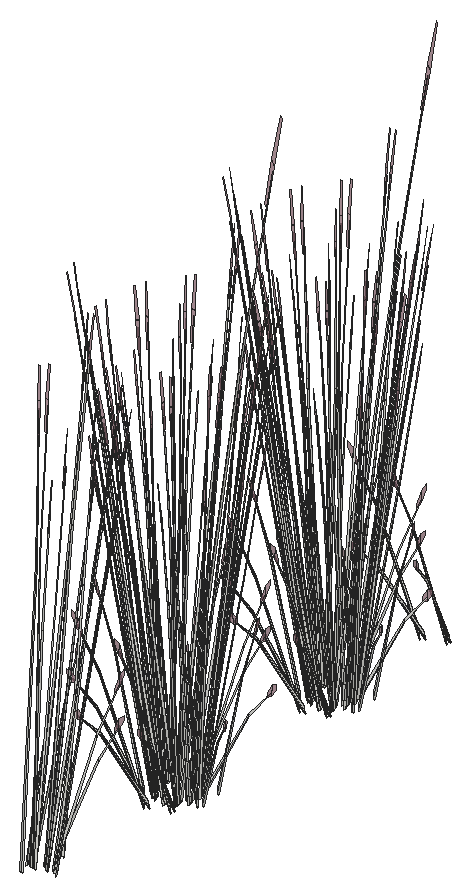
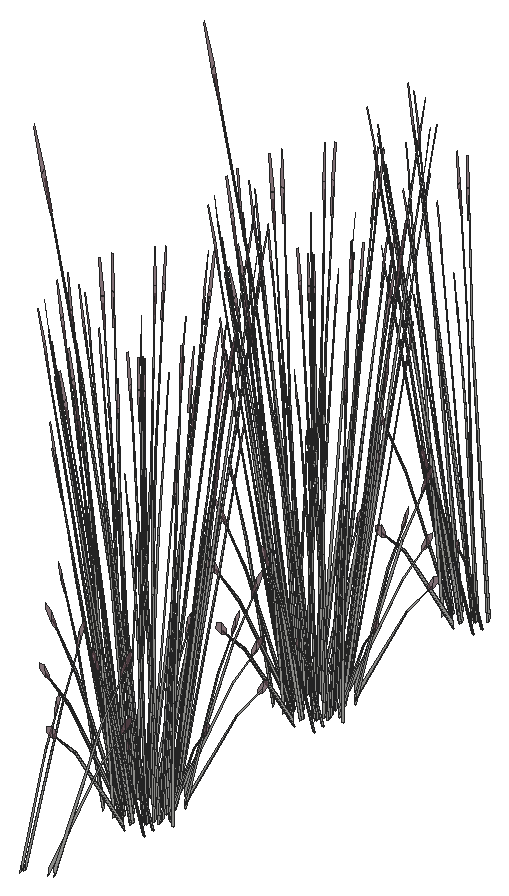
# SketchUp Ruby script. Lengths in inches.
U = 1.inch
M = Sketchup.active_model
def pt(a) = Geom::Point3d.new(a.map { |v| v * U })
def face(e, loops, mat)
  f = e.add_face(loops[0].map { |a| pt(a) })
  loops[1..].each { |l| e.add_face(l.map { |a| pt(a) }).erase! }
  f.material = f.back_material = mat if mat
  f
end
# faces: each face lists its corners as indices into pts; further lists are holes
def faces(e, pts, list, mat = nil) = list.each { |f| face(e, (f[0].is_a?(Array) ? f : [f]).map { |l| l.map { |i| pts[i] } }, mat) }
# xy, xz, yz: faces in a plane at the given z, y or x. An outline is a flat list of corners, or four numbers for a rectangle; further outlines are holes
def ring(l) = l.size == 4 ? [[l[0], l[1]], [l[2], l[1]], [l[2], l[3]], [l[0], l[3]]] : l.each_slice(2).to_a
def flat(e, list, mat, &to3) = list.each { |f| face(e, (f[0].is_a?(Array) ? f : [f]).map { |l| ring(l).map { |u, v| to3.(u, v) } }, mat) }
def xy(e, z, list, mat = nil) = flat(e, list, mat) { |x, y| [x, y, z] }
def xz(e, y, list, mat = nil) = flat(e, list, mat) { |x, z| [x, y, z] }
def yz(e, x, list, mat = nil) = flat(e, list, mat) { |y, z| [x, y, z] }
def lines(e, pts, list) = list.each { |a, b| e.add_line(pt(pts[a]), pt(pts[b])) }
# prism: a flat outline (further loops are holes) pulled along v
def prism(e, loops, v, mat = nil)
  f = face(e, loops, mat); d = Geom::Vector3d.new(v.map { |x| x * U })
  f.pushpull(f.normal.samedirection?(d) ? d.length : -d.length)
end
def box(e, o, s, mat = nil) = prism(e, [[o, [o[0] + s[0], o[1], o[2]], [o[0] + s[0], o[1] + s[1], o[2]], [o[0], o[1] + s[1], o[2]]]], [0, 0, s[2]], mat)
def at(x, y, z, deg = 0) = Geom::Transformation.translation(pt([x, y, z])) * Geom::Transformation.rotation(ORIGIN, Z_AXIS, deg.degrees)
def axes(o, x, y, z) = Geom::Transformation.new([*x, 0, *y, 0, *z, 0, *pt(o).to_a, 1])
def part(name) = M.definitions.add(name)
# library, detail: a bought-in or finely detailed component or shape, given as its bounding box
def library(name, o, s) = part(name).tap { |d| box(d.entities, o, s) }
def detail(e, o, s) = box(e.add_group.entities, o, s)
def put(e, d, t, mat = nil) = e.add_instance(d, t).tap { |i| i.material = mat if mat }
def group(e, t, mat = nil) = e.add_group.tap { |g| g.transformation = t; g.material = mat if mat }.entities
root = M.entities
M.materials.add("LightPink_Translucent").color = [144, 107, 117]
M.materials["LightPink_Translucent"].alpha = 0.75
c1 = part("blade")
p = [[2.15,0.21,22],[0,0.17,0],[0.09,0.45,0],[2.18,0.31,22],[2.29,0.31,22],[0.38,0.45,0],
  [2.48,0.24,33],[2.49,0.24,33],[2.48,0.22,33]]
faces(c1.entities,p,[[0,1,2,3],[4,5,2,3],[6,3,4,7],[8,0,3,6]])
c2 = part("seeds")
p = [[0.3,-0.1,1.38],[-0.01,-0.03,1.59],[-0.01,-0.03,0.03],[0.14,-0.07,-0.07],[0.29,-0.03,3],[0.15,0.01,3.11]]
faces(c2.entities,p,[[0,1,2,3],[1,0,4,5]],"LightPink_Translucent")
c3 = part("blade with seeds")
put(c3.entities,c1,at(0,0,0))
put(c3.entities,c2,axes([2.4,0.25,30.99],[1.5799,-0.05474,1.17369],[-0.12525,1.92788,0.29478],[-0.07173,-0.02425,1.56792]))
put(root,c3,axes([400.53,708.79,5.03],[0.32648,0.25715,-0.1216],[-0.18809,0.3724,-0.67495],[-0.09224,0.12945,1.02557]))
put(root,c3,axes([402.49,710.13,5.03],[0.21031,-0.39918,-0.1216],[0.30457,0.22997,-0.67495],[0.10587,0.11278,1.02557]))
put(root,c3,axes([401.1,709.59,5.05],[0.23881,-0.24554,0.35414],[0.22606,0.28036,-0.4572],[-0.0344,0.14245,0.87481]))
put(root,c3,axes([402.21,710.46,4.71],[0.00104,-0.05646,1.77383],[0.30246,-0.2491,-0.16761],[0.10506,0.08891,0.31391]))
put(root,c3,axes([400.88,709.8125,4.73],[-0.29004,-0.02173,0.0643],[0.00795,-0.32812,0.50621],[-0.03035,0.12569,0.77189]))
put(root,c3,axes([400.98,709.84,4.73],[-0.25132,-0.3182,0.48003],[0.2669,-0.27442,0.3958],[-0.04636,0.14929,0.9933]))
put(root,c3,axes([401.77,709.99,5.05],[0.1064,-0.35863,0.35414],[0.31043,0.1046,-0.4572],[0.02846,0.14439,0.87481]))
put(root,c3,axes([402.56,710.27,4.73],[-0.16041,0.29625,0.0643],[-0.22843,-0.17248,0.50621],[0.07385,0.09498,0.77189]))
put(root,c3,axes([402.1875,711.27,5.65],[0.2439,-0.26754,-0.06488],[0.22348,0.29302,-0.29416],[0.01573,0.08303,0.97024]))
put(root,c3,axes([402.63,710.19,4.73],[-0.35104,0.10702,0.48003],[-0.06092,-0.41983,0.3958],[0.08256,0.12373,0.9933]))
put(root,c3,axes([401.67,710.32,4.73],[-0.26007,0.1585,0.0643],[-0.12729,-0.28902,0.50621],[0.02512,0.1274,0.77189]))
put(root,c3,axes([400.15,709.86,4.72],[-0.00877,0.09229,1.74944],[0.24897,0.32105,-0.27667],[-0.06518,0.15182,0.14031]))
put(root,c3,axes([400.95,709.66,5.4],[0.3879,0.02311,-0.13498],[-0.0106,0.43749,-0.74919],[-0.02694,0.1685,1.13838]))
put(root,c3,axes([401.67,710.14,5.03],[0.34538,-0.21713,-0.1216],[0.16972,0.38536,-0.67495],[0.04557,0.16239,1.02557]))
put(root,c3,axes([401.77,710.29,5.0625],[-0.34777,-0.12192,0.53283],[0.11892,-0.40083,0.43934],[0.0209,0.15763,1.10256]))
put(root,c3,axes([400.125,710.81,4.71],[0.04004,-0.02816,1.77383],[0.33095,0.18728,-0.16761],[-0.00778,0.15594,0.31391]))
put(root,c3,axes([401.58,711.01,4.72],[0.04474,0.0751,1.74944],[0.36104,0.0295,-0.27667],[0.03631,0.16562,0.14031]))
put(root,c3,axes([401.89,721.48,4.72],[-0.05398,-0.06539,1.74944],[-0.36026,0.04145,-0.27667],[-0.0575,-0.15639,0.14031]))
put(root,c3,axes([403.51,722.29,4.72],[-0.00341,-0.09282,1.74944],[-0.28775,-0.26825,-0.27667],[0.04449,-0.16261,0.14031]))
put(root,c3,axes([403.43,721.95,4.71],[-0.03584,0.03562,1.77383],[-0.35118,-0.12018,-0.16761],[-0.01271,-0.15545,0.31391]))
put(root,c3,axes([401.52,721.27,4.71],[-0.00658,0.0559,1.77383],[-0.32474,0.20287,-0.16761],[-0.09556,-0.1037,0.31391]))
put(root,c3,axes([401.45,722.26,5.09],[0.39316,-0.11987,0.53763],[0.06823,0.47021,0.4433],[-0.09247,-0.13858,1.11249]))
put(root,c3,axes([402.34,722.35,4.73],[0.34777,0.12192,0.48003],[-0.11892,0.40083,0.3958],[-0.0209,-0.15763,0.9933]))
put(root,c3,axes([402.4375,722.49,5.03],[-0.34538,0.21713,-0.1216],[-0.16972,-0.38536,-0.67495],[-0.04557,-0.16239,1.02557]))
put(root,c3,axes([403.15,722.98,5.03],[-0.3879,-0.02311,-0.1216],[0.0106,-0.43749,-0.67495],[0.02694,-0.1685,1.02557]))
put(root,c3,axes([402.43,722.32,4.73],[0.26007,-0.1585,0.0643],[0.12729,0.28902,0.50621],[-0.02512,-0.1274,0.77189]))
put(root,c3,axes([401.54,722.36,4.73],[0.16041,-0.29625,0.0643],[0.22843,0.17248,0.50621],[-0.07385,-0.09498,0.77189]))
put(root,c3,axes([402.33,722.64,5.05],[-0.1064,0.35863,0.35414],[-0.31043,-0.1046,-0.4572],[-0.02846,-0.14439,0.87481]))
put(root,c3,axes([403.125,722.8,4.73],[0.25132,0.3182,0.48003],[-0.2669,0.27442,0.3958],[0.04636,-0.14929,0.9933]))
put(root,c3,axes([401.61,722.33,5.43],[-0.23555,0.44708,-0.13619],[-0.34112,-0.25757,-0.75594],[-0.11858,-0.12631,1.14864]))
put(root,c3,axes([403.22,722.83,4.73],[0.29004,0.02173,0.0643],[-0.00795,0.32812,0.50621],[0.03035,-0.12569,0.77189]))
put(root,c3,axes([403,723.05,5.05],[-0.23881,0.24554,0.35414],[-0.22606,-0.28036,-0.4572],[0.0344,-0.14245,0.87481]))
put(root,c3,axes([400.71,722.2,4.72],[-0.07594,-0.00329,1.74944],[-0.24177,0.32918,-0.27667],[-0.129,-0.06726,0.14031]))
put(root,c3,axes([403.58,723.84,5.03],[-0.32648,-0.25715,-0.1216],[0.18809,-0.3724,-0.67495],[0.09224,-0.12945,1.02557]))
put(root,c3,axes([401.59,722.7,5.05],[0.05451,0.37564,0.35414],[-0.31161,0.09919,-0.4572],[-0.0837,-0.10765,0.87481]))
put(root,c3,axes([400.65,722.95,5.09],[0.29147,-0.34417,0.53763],[0.25138,0.3655,0.4433],[-0.13675,-0.06349,1.11249]))
put(root,c3,axes([404.38,723.73,4.71],[-0.0461,-0.00354,1.77383],[-0.19143,-0.37951,-0.16761],[0.07688,-0.12478,0.31391]))
put(root,c3,axes([400.78,722.95,4.73],[0.01777,-0.35463,0.0643],[0.26836,0.00972,0.50621],[-0.1028,-0.03711,0.77189]))
put(root,c3,axes([403.42,723.81,5.05],[-0.30722,0.06665,0.35414],[-0.08112,-0.381,-0.4572],[0.08804,-0.10234,0.87481]))
put(root,c3,axes([403.7,723.75,4.73],[0.2423,0.19613,0.0643],[-0.14107,0.2793,0.50621],[0.07768,-0.0903,0.77189]))
put(root,c3,axes([403.63,723.66,4.73],[0.08753,0.42921,0.48003],[-0.34336,0.07449,0.3958],[0.1012,-0.10094,0.9933]))
put(root,c3,axes([404.55,724.18,4.72],[0.04898,-0.07104,1.74944],[-0.06269,-0.43574,-0.27667],[0.12289,-0.08262,0.14031]))
put(root,c3,axes([400.42,722.48,4.71],[0.02617,0.04654,1.77383],[-0.12614,0.41836,-0.16761],[-0.12775,0.00303,0.31391]))
put(root,c3,axes([400.97,723.21,5.05],[0.20082,0.29199,0.35414],[-0.2293,0.2764,-0.4572],[-0.1165,-0.04206,0.87481]))
put(root,c3,axes([400.91,723.02,5.03],[-0.0189,0.47427,-0.1216],[-0.35781,-0.01296,-0.67495],[-0.13781,-0.03295,1.02557]))
put(root,c3,axes([403.59,724.85,5.03],[-0.17758,-0.42229,-0.1216],[0.31518,-0.20752,-0.67495],[0.13282,-0.05572,1.02557]))
put(root,c3,axes([403.47,724.72,5.05],[-0.29332,-0.1301,0.35414],[0.08555,-0.37955,-0.4572],[0.11809,-0.0348,0.87481]))
put(root,c3,axes([400.4,724.02,4.73],[0.09971,-0.42522,0.48003],[0.32782,0.1454,0.3958],[-0.12892,0.02555,0.9933]))
put(root,c3,axes([400.37,723.91,4.73],[-0.12963,-0.31798,0.0643],[0.23638,-0.15564,0.50621],[-0.1042,0.03071,0.77189]))
put(root,c3,axes([403.73,724.84,4.73],[0.12963,0.31798,0.0643],[-0.23638,0.15564,0.50621],[0.1042,-0.03071,0.77189]))
put(root,c3,axes([403.71,724.72,4.73],[-0.09971,0.42522,0.48003],[-0.32782,-0.1454,0.3958],[0.12892,-0.02555,0.9933]))
put(root,c3,axes([400.64,724.03,5.05],[0.29332,0.1301,0.35414],[-0.08555,0.37955,-0.4572],[-0.11809,0.0348,0.87481]))
put(root,c3,axes([404.3,726.1,4.71],[-0.03191,-0.04083,1.77383],[0.06981,-0.43764,-0.16761],[0.12571,-0.02796,0.31391]))
put(root,c3,axes([400.14,724.32,4.72],[-0.05763,0.06055,1.74944],[0.0049,0.44239,-0.27667],[-0.13211,0.05753,0.14031]))
put(root,c3,axes([400.51,723.9,5.03],[0.17758,0.42229,-0.1216],[-0.31518,0.20752,-0.67495],[-0.13282,0.05572,1.02557]))
put(root,c3,axes([403.19,725.72,5.03],[0.0189,-0.47427,-0.1216],[0.35781,0.01296,-0.67495],[0.13781,0.03295,1.02557]))
put(root,c3,axes([403.14,725.54,5.05],[-0.20082,-0.29199,0.35414],[0.2293,-0.2764,-0.4572],[0.1165,0.04206,0.87481]))
put(root,c3,axes([403.5,725.4375,4.72],[0.07571,-0.00789,1.74944],[0.20767,-0.36231,-0.27667],[0.13467,0.04783,0.14031]))
put(root,c3,axes([400.47,725.08,4.73],[-0.08753,-0.42921,0.48003],[0.34336,-0.07449,0.3958],[-0.1012,0.10094,0.9933]))
put(root,c3,axes([400.41,725,4.73],[-0.2423,-0.19613,0.0643],[0.14107,-0.2793,0.50621],[-0.07768,0.0903,0.77189]))
put(root,c3,axes([400.6875,724.94,5.05],[0.30722,-0.06665,0.35414],[0.08112,0.381,-0.4572],[-0.08804,0.10234,0.87481]))
put(root,c3,axes([399.5,724.77,4.71],[0.04504,0.01251,1.77383],[0.13934,0.41205,-0.16761],[-0.0922,0.10815,0.31391]))
put(root,c3,axes([403.32,725.8,4.73],[-0.01777,0.35463,0.0643],[-0.26836,-0.00972,0.50621],[0.1028,0.03711,0.77189]))
put(root,c3,axes([403.34,725.6875,4.73],[-0.26024,0.30729,0.48003],[-0.22444,-0.32634,0.3958],[0.1221,0.05668,0.9933]))
put(root,c3,axes([399.99,726.02,5.65],[0.31145,0.12449,-0.06488],[-0.0958,0.38314,-0.29416],[-0.05094,0.05817,0.97024]))
put(root,c3,axes([402.52,726.04,5.05],[-0.05451,-0.37564,0.35414],[0.31161,-0.09919,-0.4572],[0.0837,0.10765,0.87481]))
put(root,c3,axes([402.72,723.88,4.47],[-0.30498,-0.24231,1.38283],[0.32203,-0.37727,0.59665],[0.0984,0.22736,1.33663]))
put(root,c3,axes([400.53,724.91,5.03],[0.32648,0.25715,-0.1216],[-0.18809,0.3724,-0.67495],[-0.09224,0.12945,1.02557]))
put(root,c3,axes([402.49,726.24,5.03],[0.21031,-0.39918,-0.1216],[0.30457,0.22997,-0.67495],[0.10587,0.11278,1.02557]))
put(root,c3,axes([401.1,725.7,5.05],[0.23881,-0.24554,0.35414],[0.22606,0.28036,-0.4572],[-0.0344,0.14245,0.87481]))
put(root,c3,axes([402.21,726.57,4.71],[0.00104,-0.05646,1.77383],[0.30246,-0.2491,-0.16761],[0.10506,0.08891,0.31391]))
put(root,c3,axes([400.88,725.92,4.73],[-0.29004,-0.02173,0.0643],[0.00795,-0.32812,0.50621],[-0.03035,0.12569,0.77189]))
put(root,c3,axes([400.98,725.95,4.73],[-0.25132,-0.3182,0.48003],[0.2669,-0.27442,0.3958],[-0.04636,0.14929,0.9933]))
put(root,c3,axes([401.77,726.1,5.05],[0.1064,-0.35863,0.35414],[0.31043,0.1046,-0.4572],[0.02846,0.14439,0.87481]))
put(root,c3,axes([402.56,726.38,4.73],[-0.16041,0.29625,0.0643],[-0.22843,-0.17248,0.50621],[0.07385,0.09498,0.77189]))
put(root,c3,axes([402.1875,727.38,5.65],[0.2439,-0.26754,-0.06488],[0.22348,0.29302,-0.29416],[0.01573,0.08303,0.97024]))
put(root,c3,axes([402.63,726.3,4.73],[-0.35104,0.10702,0.48003],[-0.06092,-0.41983,0.3958],[0.08256,0.12373,0.9933]))
put(root,c3,axes([401.67,726.43,4.73],[-0.26007,0.1585,0.0643],[-0.12729,-0.28902,0.50621],[0.02512,0.1274,0.77189]))
put(root,c3,axes([400.15,725.98,4.72],[-0.00877,0.09229,1.74944],[0.24897,0.32105,-0.27667],[-0.06518,0.15182,0.14031]))
put(root,c3,axes([400.95,725.77,5.4],[0.3879,0.02311,-0.13498],[-0.0106,0.43749,-0.74919],[-0.02694,0.1685,1.13838]))
put(root,c3,axes([401.67,726.25,5.03],[0.34538,-0.21713,-0.1216],[0.16972,0.38536,-0.67495],[0.04557,0.16239,1.02557]))
put(root,c3,axes([401.77,726.4,5.0625],[-0.34777,-0.12192,0.53283],[0.11892,-0.40083,0.43934],[0.0209,0.15763,1.10256]))
put(root,c3,axes([400.125,726.92,4.71],[0.04004,-0.02816,1.77383],[0.33095,0.18728,-0.16761],[-0.00778,0.15594,0.31391]))
put(root,c3,axes([401.58,727.12,4.72],[0.04474,0.0751,1.74944],[0.36104,0.0295,-0.27667],[0.03631,0.16562,0.14031]))
put(root,c3,axes([401.89,738.63,4.72],[-0.05398,-0.06539,1.74944],[-0.36026,0.04145,-0.27667],[-0.0575,-0.15639,0.14031]))
put(root,c3,axes([403.51,739.43,4.72],[-0.00341,-0.09282,1.74944],[-0.28775,-0.26825,-0.27667],[0.04449,-0.16261,0.14031]))
put(root,c3,axes([403.43,739.1,4.71],[-0.03584,0.03562,1.77383],[-0.35118,-0.12018,-0.16761],[-0.01271,-0.15545,0.31391]))
put(root,c3,axes([401.52,738.42,4.71],[-0.00658,0.0559,1.77383],[-0.32474,0.20287,-0.16761],[-0.09556,-0.1037,0.31391]))
put(root,c3,axes([401.45,739.41,5.09],[0.39316,-0.11987,0.53763],[0.06823,0.47021,0.4433],[-0.09247,-0.13858,1.11249]))
put(root,c3,axes([402.34,739.5,4.73],[0.34777,0.12192,0.48003],[-0.11892,0.40083,0.3958],[-0.0209,-0.15763,0.9933]))
put(root,c3,axes([402.4375,739.64,5.03],[-0.34538,0.21713,-0.1216],[-0.16972,-0.38536,-0.67495],[-0.04557,-0.16239,1.02557]))
put(root,c3,axes([403.15,740.125,5.03],[-0.3879,-0.02311,-0.1216],[0.0106,-0.43749,-0.67495],[0.02694,-0.1685,1.02557]))
put(root,c3,axes([402.43,739.47,4.73],[0.26007,-0.1585,0.0643],[0.12729,0.28902,0.50621],[-0.02512,-0.1274,0.77189]))
put(root,c3,axes([401.54,739.51,4.73],[0.16041,-0.29625,0.0643],[0.22843,0.17248,0.50621],[-0.07385,-0.09498,0.77189]))
put(root,c3,axes([402.33,739.79,5.05],[-0.1064,0.35863,0.35414],[-0.31043,-0.1046,-0.4572],[-0.02846,-0.14439,0.87481]))
put(root,c3,axes([403.125,739.94,4.73],[0.25132,0.3182,0.48003],[-0.2669,0.27442,0.3958],[0.04636,-0.14929,0.9933]))
put(root,c3,axes([401.61,739.48,5.43],[-0.23555,0.44708,-0.13619],[-0.34112,-0.25757,-0.75594],[-0.11858,-0.12631,1.14864]))
put(root,c3,axes([403.22,739.97,4.73],[0.29004,0.02173,0.0643],[-0.00795,0.32812,0.50621],[0.03035,-0.12569,0.77189]))
put(root,c3,axes([403,740.19,5.05],[-0.23881,0.24554,0.35414],[-0.22606,-0.28036,-0.4572],[0.0344,-0.14245,0.87481]))
put(root,c3,axes([400.71,739.35,4.72],[-0.07594,-0.00329,1.74944],[-0.24177,0.32918,-0.27667],[-0.129,-0.06726,0.14031]))
put(root,c3,axes([403.58,740.99,5.03],[-0.32648,-0.25715,-0.1216],[0.18809,-0.3724,-0.67495],[0.09224,-0.12945,1.02557]))
put(root,c3,axes([401.59,739.85,5.05],[0.05451,0.37564,0.35414],[-0.31161,0.09919,-0.4572],[-0.0837,-0.10765,0.87481]))
put(root,c3,axes([400.65,740.09,5.09],[0.29147,-0.34417,0.53763],[0.25138,0.3655,0.4433],[-0.13675,-0.06349,1.11249]))
put(root,c3,axes([404.38,740.875,4.71],[-0.0461,-0.00354,1.77383],[-0.19143,-0.37951,-0.16761],[0.07688,-0.12478,0.31391]))
put(root,c3,axes([400.78,740.09,4.73],[0.01777,-0.35463,0.0643],[0.26836,0.00972,0.50621],[-0.1028,-0.03711,0.77189]))
put(root,c3,axes([403.42,740.95,5.05],[-0.30722,0.06665,0.35414],[-0.08112,-0.381,-0.4572],[0.08804,-0.10234,0.87481]))
put(root,c3,axes([403.7,740.89,4.73],[0.2423,0.19613,0.0643],[-0.14107,0.2793,0.50621],[0.07768,-0.0903,0.77189]))
put(root,c3,axes([403.63,740.81,4.73],[0.08753,0.42921,0.48003],[-0.34336,0.07449,0.3958],[0.1012,-0.10094,0.9933]))
put(root,c3,axes([404.55,741.33,4.72],[0.04898,-0.07104,1.74944],[-0.06269,-0.43574,-0.27667],[0.12289,-0.08262,0.14031]))
put(root,c3,axes([400.42,739.63,4.71],[0.02617,0.04654,1.77383],[-0.12614,0.41836,-0.16761],[-0.12775,0.00303,0.31391]))
put(root,c3,axes([400.97,740.36,5.05],[0.20082,0.29199,0.35414],[-0.2293,0.2764,-0.4572],[-0.1165,-0.04206,0.87481]))
put(root,c3,axes([400.91,740.17,5.03],[-0.0189,0.47427,-0.1216],[-0.35781,-0.01296,-0.67495],[-0.13781,-0.03295,1.02557]))
put(root,c3,axes([403.59,741.99,5.03],[-0.17758,-0.42229,-0.1216],[0.31518,-0.20752,-0.67495],[0.13282,-0.05572,1.02557]))
put(root,c3,axes([403.47,741.86,5.05],[-0.29332,-0.1301,0.35414],[0.08555,-0.37955,-0.4572],[0.11809,-0.0348,0.87481]))
put(root,c3,axes([400.4,741.17,4.73],[0.09971,-0.42522,0.48003],[0.32782,0.1454,0.3958],[-0.12892,0.02555,0.9933]))
put(root,c3,axes([400.37,741.06,4.73],[-0.12963,-0.31798,0.0643],[0.23638,-0.15564,0.50621],[-0.1042,0.03071,0.77189]))
put(root,c3,axes([403.73,741.98,4.73],[0.12963,0.31798,0.0643],[-0.23638,0.15564,0.50621],[0.1042,-0.03071,0.77189]))
put(root,c3,axes([403.71,741.87,4.73],[-0.09971,0.42522,0.48003],[-0.32782,-0.1454,0.3958],[0.12892,-0.02555,0.9933]))
put(root,c3,axes([400.64,741.18,5.05],[0.29332,0.1301,0.35414],[-0.08555,0.37955,-0.4572],[-0.11809,0.0348,0.87481]))
put(root,c3,axes([404.3,743.25,4.71],[-0.03191,-0.04083,1.77383],[0.06981,-0.43764,-0.16761],[0.12571,-0.02796,0.31391]))
put(root,c3,axes([400.14,741.47,4.72],[-0.05763,0.06055,1.74944],[0.0049,0.44239,-0.27667],[-0.13211,0.05753,0.14031]))
put(root,c3,axes([400.51,741.05,5.03],[0.17758,0.42229,-0.1216],[-0.31518,0.20752,-0.67495],[-0.13282,0.05572,1.02557]))
put(root,c3,axes([403.19,742.87,5.03],[0.0189,-0.47427,-0.1216],[0.35781,0.01296,-0.67495],[0.13781,0.03295,1.02557]))
put(root,c3,axes([403.14,742.68,5.05],[-0.20082,-0.29199,0.35414],[0.2293,-0.2764,-0.4572],[0.1165,0.04206,0.87481]))
put(root,c3,axes([403.5,742.58,4.72],[0.07571,-0.00789,1.74944],[0.20767,-0.36231,-0.27667],[0.13467,0.04783,0.14031]))
put(root,c3,axes([400.47,742.23,4.73],[-0.08753,-0.42921,0.48003],[0.34336,-0.07449,0.3958],[-0.1012,0.10094,0.9933]))
put(root,c3,axes([400.41,742.15,4.73],[-0.2423,-0.19613,0.0643],[0.14107,-0.2793,0.50621],[-0.07768,0.0903,0.77189]))
put(root,c3,axes([400.6875,742.09,5.05],[0.30722,-0.06665,0.35414],[0.08112,0.381,-0.4572],[-0.08804,0.10234,0.87481]))
put(root,c3,axes([399.5,741.92,4.71],[0.04504,0.01251,1.77383],[0.13934,0.41205,-0.16761],[-0.0922,0.10815,0.31391]))
put(root,c3,axes([403.32,742.95,4.73],[-0.01777,0.35463,0.0643],[-0.26836,-0.00972,0.50621],[0.1028,0.03711,0.77189]))
put(root,c3,axes([403.34,742.83,4.73],[-0.26024,0.30729,0.48003],[-0.22444,-0.32634,0.3958],[0.1221,0.05668,0.9933]))
put(root,c3,axes([399.99,743.17,5.65],[0.31145,0.12449,-0.06488],[-0.0958,0.38314,-0.29416],[-0.05094,0.05817,0.97024]))
put(root,c3,axes([402.52,743.19,5.05],[-0.05451,-0.37564,0.35414],[0.31161,-0.09919,-0.4572],[0.0837,0.10765,0.87481]))
put(root,c3,axes([402.72,741.03,4.47],[-0.30498,-0.24231,1.38283],[0.32203,-0.37727,0.59665],[0.0984,0.22736,1.33663]))
put(root,c3,axes([400.53,742.05,5.03],[0.32648,0.25715,-0.1216],[-0.18809,0.3724,-0.67495],[-0.09224,0.12945,1.02557]))
put(root,c3,axes([402.49,743.38,5.03],[0.21031,-0.39918,-0.1216],[0.30457,0.22997,-0.67495],[0.10587,0.11278,1.02557]))
put(root,c3,axes([401.1,742.85,5.05],[0.23881,-0.24554,0.35414],[0.22606,0.28036,-0.4572],[-0.0344,0.14245,0.87481]))
put(root,c3,axes([402.21,743.72,4.71],[0.00104,-0.05646,1.77383],[0.30246,-0.2491,-0.16761],[0.10506,0.08891,0.31391]))
put(root,c3,axes([400.88,743.07,4.73],[-0.29004,-0.02173,0.0643],[0.00795,-0.32812,0.50621],[-0.03035,0.12569,0.77189]))
put(root,c3,axes([400.98,743.1,4.73],[-0.25132,-0.3182,0.48003],[0.2669,-0.27442,0.3958],[-0.04636,0.14929,0.9933]))
put(root,c3,axes([401.77,743.25,5.05],[0.1064,-0.35863,0.35414],[0.31043,0.1046,-0.4572],[0.02846,0.14439,0.87481]))
put(root,c3,axes([402.56,743.53,4.73],[-0.16041,0.29625,0.0643],[-0.22843,-0.17248,0.50621],[0.07385,0.09498,0.77189]))
put(root,c3,axes([402.1875,744.53,5.65],[0.2439,-0.26754,-0.06488],[0.22348,0.29302,-0.29416],[0.01573,0.08303,0.97024]))
put(root,c3,axes([402.63,743.45,4.73],[-0.35104,0.10702,0.48003],[-0.06092,-0.41983,0.3958],[0.08256,0.12373,0.9933]))
put(root,c3,axes([401.67,743.58,4.73],[-0.26007,0.1585,0.0643],[-0.12729,-0.28902,0.50621],[0.02512,0.1274,0.77189]))
put(root,c3,axes([400.15,743.12,4.72],[-0.00877,0.09229,1.74944],[0.24897,0.32105,-0.27667],[-0.06518,0.15182,0.14031]))
put(root,c3,axes([400.95,742.91,5.4],[0.3879,0.02311,-0.13498],[-0.0106,0.43749,-0.74919],[-0.02694,0.1685,1.13838]))
put(root,c3,axes([401.67,743.4,5.03],[0.34538,-0.21713,-0.1216],[0.16972,0.38536,-0.67495],[0.04557,0.16239,1.02557]))
put(root,c3,axes([401.77,743.54,5.0625],[-0.34777,-0.12192,0.53283],[0.11892,-0.40083,0.43934],[0.0209,0.15763,1.10256]))
put(root,c3,axes([400.125,744.07,4.71],[0.04004,-0.02816,1.77383],[0.33095,0.18728,-0.16761],[-0.00778,0.15594,0.31391]))
put(root,c3,axes([401.58,744.26,4.72],[0.04474,0.0751,1.74944],[0.36104,0.0295,-0.27667],[0.03631,0.16562,0.14031]))
put(root,c3,axes([401.89,751.86,4.72],[-0.05398,-0.06539,1.74944],[-0.36026,0.04145,-0.27667],[-0.0575,-0.15639,0.14031]))
put(root,c3,axes([403.51,752.66,4.72],[-0.00341,-0.09282,1.74944],[-0.28775,-0.26825,-0.27667],[0.04449,-0.16261,0.14031]))
put(root,c3,axes([403.43,752.33,4.71],[-0.03584,0.03562,1.77383],[-0.35118,-0.12018,-0.16761],[-0.01271,-0.15545,0.31391]))
put(root,c3,axes([401.52,751.65,4.71],[-0.00658,0.0559,1.77383],[-0.32474,0.20287,-0.16761],[-0.09556,-0.1037,0.31391]))
